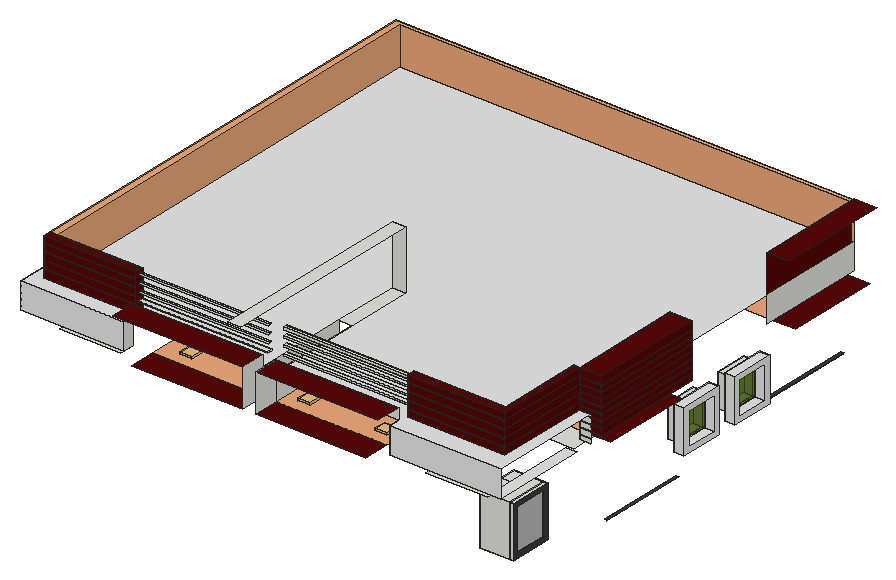
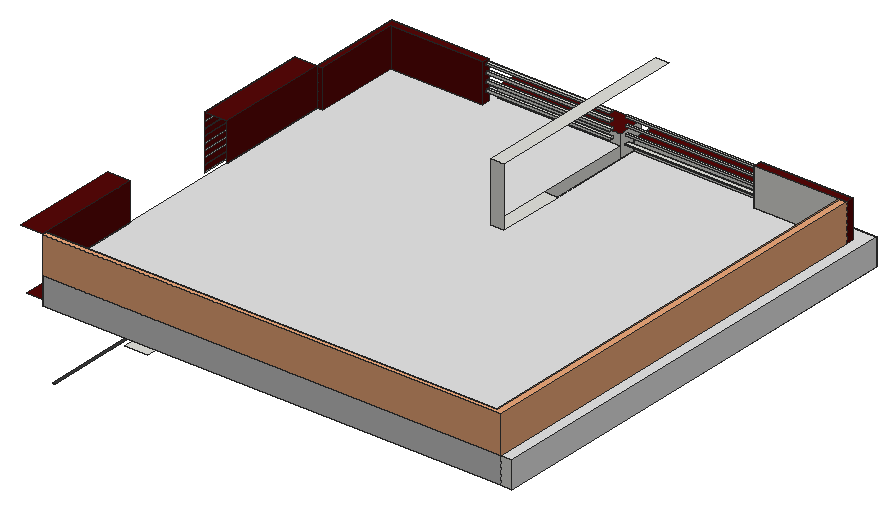
# SketchUp Ruby script. Lengths in inches.
U = 1.inch
M = Sketchup.active_model
def pt(a) = Geom::Point3d.new(a.map { |v| v * U })
def face(e, loops, mat)
  f = e.add_face(loops[0].map { |a| pt(a) })
  loops[1..].each { |l| e.add_face(l.map { |a| pt(a) }).erase! }
  f.material = f.back_material = mat if mat
  f
end
# faces: each face lists its corners as indices into pts; further lists are holes
def faces(e, pts, list, mat = nil) = list.each { |f| face(e, (f[0].is_a?(Array) ? f : [f]).map { |l| l.map { |i| pts[i] } }, mat) }
# xy, xz, yz: faces in a plane at the given z, y or x. An outline is a flat list of corners, or four numbers for a rectangle; further outlines are holes
def ring(l) = l.size == 4 ? [[l[0], l[1]], [l[2], l[1]], [l[2], l[3]], [l[0], l[3]]] : l.each_slice(2).to_a
def flat(e, list, mat, &to3) = list.each { |f| face(e, (f[0].is_a?(Array) ? f : [f]).map { |l| ring(l).map { |u, v| to3.(u, v) } }, mat) }
def xy(e, z, list, mat = nil) = flat(e, list, mat) { |x, y| [x, y, z] }
def xz(e, y, list, mat = nil) = flat(e, list, mat) { |x, z| [x, y, z] }
def yz(e, x, list, mat = nil) = flat(e, list, mat) { |y, z| [x, y, z] }
def lines(e, pts, list) = list.each { |a, b| e.add_line(pt(pts[a]), pt(pts[b])) }
# prism: a flat outline (further loops are holes) pulled along v
def prism(e, loops, v, mat = nil)
  f = face(e, loops, mat); d = Geom::Vector3d.new(v.map { |x| x * U })
  f.pushpull(f.normal.samedirection?(d) ? d.length : -d.length)
end
def box(e, o, s, mat = nil) = prism(e, [[o, [o[0] + s[0], o[1], o[2]], [o[0] + s[0], o[1] + s[1], o[2]], [o[0], o[1] + s[1], o[2]]]], [0, 0, s[2]], mat)
def at(x, y, z, deg = 0) = Geom::Transformation.translation(pt([x, y, z])) * Geom::Transformation.rotation(ORIGIN, Z_AXIS, deg.degrees)
def axes(o, x, y, z) = Geom::Transformation.new([*x, 0, *y, 0, *z, 0, *pt(o).to_a, 1])
def part(name) = M.definitions.add(name)
# library, detail: a bought-in or finely detailed component or shape, given as its bounding box
def library(name, o, s) = part(name).tap { |d| box(d.entities, o, s) }
def detail(e, o, s) = box(e.add_group.entities, o, s)
def put(e, d, t, mat = nil) = e.add_instance(d, t).tap { |i| i.material = mat if mat }
def group(e, t, mat = nil) = e.add_group.tap { |g| g.transformation = t; g.material = mat if mat }.entities
root = M.entities
M.materials.add("Generic").color = [86, 8, 8]
M.materials.add("Generic\#1").color = [236, 168, 122]
M.materials.add("Generic\#4").color = [201, 201, 201]
M.materials.add("Generic\#5").color = [230, 230, 230]
M.materials.add("[Color M07]").color = [58, 58, 58]
M.materials.add("[Mirror 01]").color = [185, 185, 185]
M.materials.add("[Translucent Glass Dark Green]").color = [62, 91, 5]
M.materials["[Translucent Glass Dark Green]"].alpha = 0.5
c1 = part("Group\#3")
xy(c1.entities,0,[[0,0,6,62.6875]],"[Color M07]")
xy(c1.entities,6.1,[[3,6.1,6,56.59]],"[Color M07]")
xy(c1.entities,69.52,[[3,6.1,6,56.59]],"[Color M07]")
xy(c1.entities,75.625,[[0,0,6,62.6875]],"[Color M07]")
xz(c1.entities,0,[[0,0,6,75.625]],"[Color M07]")
xz(c1.entities,6.1,[[3,6.1,6,69.52]],"[Color M07]")
xz(c1.entities,56.59,[[3,6.1,6,69.52]],"[Color M07]")
xz(c1.entities,62.6875,[[0,0,6,75.625]],"[Color M07]")
yz(c1.entities,0,[[0,0,62.6875,75.625]])
yz(c1.entities,3,[[6.1,6.1,56.59,69.52]],"[Mirror 01]")
yz(c1.entities,6,[[[0,0,62.6875,75.625],[6.1,6.1,56.59,69.52]]],"[Color M07]")
c2 = part("Group\#1")
box(c2.entities,[0,0,0],[3,48.3125,48.3125],"[Translucent Glass Dark Green]")
c3 = library("Tlon Light 450 Ceiling 152 006",[-8.86,-8.86,-3.78],[17.72,17.72,3.56])
xy(root,889.17,[[648.625,141.33,698.4375,204.02]])
xy(root,891.34,[[722.32,281.625,725.7,413.625]],"[Color M07]")
xy(root,891.4375,[[688.93,624.8125,693.12,762.8125]],"[Color M07]")
xy(root,902.74,[[698.4375,439.75,713.5625,504.55]])
xy(root,902.74,[[698.4375,533.62,713.5625,598.43]],"Generic\#5")
xy(root,910.99,[[681.875,447.99,698.4375,496.3],[681.875,541.87,698.4375,590.18]])
xy(root,910.99,[[698.4375,447.99,713.5625,496.3],[698.4375,541.87,713.5625,590.18]],"Generic\#5")
xy(root,951.48,[[594.5625,306.16,656.0625,398.23]])
xy(root,959.27,[[205.11,219.4375,322.86,251.5625],[386.36,219.4375,504.11,251.5625]])
xy(root,959.3,[[681.875,447.99,698.4375,496.3],[698.4375,447.99,713.5625,496.3],[681.875,541.87,698.4375,590.18]])
xy(root,959.3,[[698.4375,541.87,713.5625,590.18]],"Generic\#5")
xy(root,964.8,[[648.625,141.33,698.4375,204.02]])
xy(root,966.4,[[563.75,654.65,598.75,746.71]])
xy(root,967.55,[[698.4375,439.75,713.5625,504.55],[698.4375,533.62,713.5625,598.43]],"Generic\#5")
xy(root,980.36,[[44.83,113.625,136.51,130.0625],[589.83,113.625,681.51,158.0625]])
xy(root,997.25,[[183.5625,219.4375,347.9375,255],[367.1875,219.4375,531.5625,255],[16.6875,762.8125,698.4375,774.8125]])
xy(root,997.25,[[183.4375,75.4375,347.9375,113.625],[367.1875,75.4375,531.6875,113.625],[698.4375,281.625,731.4375,413.625],[698.4375,624.8125,731.4375,762.8125]],"Generic")
xy(root,997.25,[[183.5625,113.625,347.9375,219.4375],[367.1875,113.625,531.5625,219.4375],[656.0625,281.625,698.4375,413.625],[598.75,624.8125,698.4375,762.8125]],"Generic\#1")
xy(root,997.25,[[0,96.5625,0,774.8125,16.6875,774.8125,16.6875,113.625,154.5,113.625,154.5,96.5625],[549.5625,96.5625,549.5625,113.625,698.4375,113.625,698.4375,238.3125,715.125,238.3125,715.125,96.5625]],"Generic\#5")
xy(root,1012.8125,[[715.125,263.625,731.4375,263.93],[731.14,263.93,731.4375,431.625]])
xy(root,1013.8125,[[715.125,263.625,731.4375,263.93],[731.14,263.93,731.4375,431.625]])
xy(root,1022.4375,[[715.125,263.625,731.4375,263.93],[731.14,263.93,731.4375,431.625]])
xy(root,1023.4375,[[715.125,263.625,731.4375,263.93],[731.14,263.93,731.4375,431.625]])
xy(root,1032.0625,[[715.125,263.625,731.4375,263.93],[731.14,263.93,731.4375,431.625]])
xy(root,1033.0625,[[715.125,263.625,731.4375,263.93],[731.14,263.93,731.4375,431.625]])
xy(root,1036.5625,[[16.6875,119.0625,154.5,131.0625],[552.85,125.625,552.85,137.625,689.4375,137.625,689.4375,263.625,698.4375,263.625,698.4375,125.625],[16.6875,131.0625,16.6875,774.8125,698.4375,774.8125,698.4375,767.9375,27.5,767.9375,27.5,131.0625],[347.9375,255,367.1875,354.125]])
xy(root,1036.5625,[[0,96.5625,154.5,96.5625,154.5,113.625,347.9375,113.625,347.9375,354.125,367.1875,354.125,367.1875,113.625,549.5625,113.625,549.5625,96.5625,715.125,96.5625,715.125,263.625,698.4375,263.625,698.4375,125.625,552.85,125.625,552.85,137.625,689.4375,137.625,689.4375,263.625,698.4375,263.625,698.4375,767.9375,27.5,767.9375,27.5,131.0625,154.5,131.0625,154.5,119.0625,16.6875,119.0625,16.6875,774.8125,0,774.8125]],"Generic\#5")
xy(root,1041.6875,[[698.4375,263.625,731.4375,263.93],[731.14,263.93,731.4375,431.625]])
xy(root,1042.6875,[[698.4375,263.625,731.4375,263.93],[731.14,263.93,731.4375,431.625]])
xy(root,1046.3125,[[552.85,125.625,698.4375,125.93],[698.14,125.93,698.4375,263.625]])
xy(root,1047.3125,[[552.85,125.625,698.4375,125.93],[698.14,125.93,698.4375,263.625]])
xy(root,1048.5625,[[16.6875,119.0625,154.5,119.36]])
xy(root,1049.5625,[[16.6875,119.0625,154.5,119.36]])
xy(root,1051.13,[[154.5,122.52,347.9375,129.9]])
xy(root,1051.3125,[[698.4375,263.625,731.4375,263.93],[731.14,263.93,731.4375,431.625]])
xy(root,1052.22,[[367.1875,126.95,552.85,132.89]])
xy(root,1052.3125,[[698.4375,263.625,731.4375,263.93],[731.14,263.93,731.4375,431.625]])
xy(root,1052.9375,[[154.5,75.4375,347.9375,113.625],[367.1875,75.4375,549.5625,113.625]],"Generic")
xy(root,1053.13,[[154.5,122.52,347.9375,129.9]])
xy(root,1055.1,[[367.1875,126.95,552.85,132.89]])
xy(root,1058.3125,[[552.85,125.625,698.14,125.93],[698.14,125.625,698.4375,263.625]])
xy(root,1059.3125,[[552.85,125.625,698.14,125.93],[698.14,125.625,698.4375,263.625]])
xy(root,1059.9375,[[16.6875,119.0625,154.5,119.36]])
xy(root,1060.9375,[[16.6875,119.0625,154.5,119.36],[698.4375,263.625,731.4375,263.93],[731.14,263.93,731.4375,431.625]])
xy(root,1061.9375,[[698.4375,263.625,731.4375,263.93],[731.14,263.93,731.4375,431.625]])
xy(root,1063.19,[[154.5,123.11,347.9375,128.18]])
xy(root,1064.22,[[367.1875,126.95,552.85,132.89]])
xy(root,1065.32,[[154.5,123.11,347.9375,128.18]])
xy(root,1067.1,[[367.1875,126.95,552.85,132.89]])
xy(root,1070.3125,[[552.85,125.625,698.4375,125.93],[698.14,125.93,698.4375,263.625]])
xy(root,1070.5625,[[698.4375,263.625,731.4375,263.93],[731.14,263.93,731.4375,431.625]])
xy(root,1071.3125,[[16.6875,119.0625,154.5,119.36],[552.85,125.625,698.4375,125.93],[698.14,125.93,698.4375,263.625]])
xy(root,1071.5625,[[698.4375,263.625,731.4375,263.93],[731.14,263.93,731.4375,431.625]])
xy(root,1072.3125,[[16.6875,119.0625,154.5,119.36]])
xy(root,1075.19,[[154.5,123.11,347.9375,128.18]])
xy(root,1076.22,[[367.1875,126.95,552.85,132.89]])
xy(root,1077.32,[[154.5,123.11,347.9375,128.18]])
xy(root,1079.1,[[367.1875,126.95,552.85,132.89]])
xy(root,1080.1875,[[698.4375,263.625,731.4375,263.93],[731.14,263.93,731.4375,431.625]])
xy(root,1081.1875,[[698.4375,263.625,731.4375,263.93],[731.14,263.93,731.4375,431.625]])
xy(root,1082.3125,[[552.85,125.625,698.14,125.93],[698.14,125.625,698.4375,263.625]])
xy(root,1082.6875,[[16.6875,119.0625,154.5,119.36]])
xy(root,1083.3125,[[552.85,125.625,698.14,125.93],[698.14,125.625,698.4375,263.625]])
xy(root,1083.6875,[[16.6875,119.0625,154.5,119.36]])
xy(root,1087.19,[[154.5,123.11,347.9375,128.18]])
xy(root,1087.4,[[367.1875,126.95,552.85,132.89]])
xy(root,1089.32,[[154.5,123.11,347.9375,128.18]])
xy(root,1090.28,[[367.1875,126.95,552.85,132.89]])
xy(root,1092.375,[[16.6875,119.0625,154.5,131.0625]],"Generic")
xy(root,1092.375,[[16.6875,131.0625,27.5,131.0625,27.5,767.9375,698.4375,767.9375,698.4375,774.8125,16.6875,774.8125]],"Generic\#1")
xy(root,1093.1875,[[552.85,125.625,698.4375,125.625,698.4375,263.625,689.4375,263.625,689.4375,137.625,552.85,137.625],[698.4375,263.625,731.4375,431.625],[698.4375,612.8125,731.4375,774.8125]],"Generic")
xy(root,1124.875,[[347.9375,48.1875,367.1875,354.125]])
xz(root,96.5625,[[0,997.25,154.5,1036.5625],[549.5625,997.25,715.125,1036.5625]],"Generic\#5")
xz(root,113.625,[[154.5,1036.5625,347.9375,1052.9375],[367.1875,1036.5625,549.5625,1052.9375]])
xz(root,119.0625,[[16.6875,1036.5625,154.5,1048.5625],[16.6875,1049.5625,154.5,1059.9375],[16.6875,1060.9375,154.5,1071.3125],[16.6875,1072.3125,154.5,1082.6875],[16.6875,1083.6875,154.5,1092.375]],"Generic")
xz(root,119.36,[[16.6875,1048.5625,154.5,1049.5625],[16.6875,1059.9375,154.5,1060.9375],[16.6875,1071.3125,154.5,1072.3125],[16.6875,1082.6875,154.5,1083.6875]])
xz(root,122.52,[[154.5,1051.13,347.9375,1053.13]])
xz(root,123.11,[[154.5,1063.19,347.9375,1065.32],[154.5,1075.19,347.9375,1077.32],[154.5,1087.19,347.9375,1089.32]])
xz(root,125.625,[[552.85,1036.5625,698.4375,1046.3125],[552.85,1047.3125,698.4375,1058.3125],[552.85,1059.3125,698.4375,1070.3125],[552.85,1071.3125,698.4375,1082.3125],[552.85,1083.3125,698.4375,1093.1875]],"Generic")
xz(root,125.93,[[552.85,1046.3125,698.14,1047.3125],[552.85,1058.3125,698.14,1059.3125],[552.85,1070.3125,698.14,1071.3125],[552.85,1082.3125,698.14,1083.3125]])
xz(root,126.95,[[367.1875,1052.22,552.85,1055.1],[367.1875,1064.22,552.85,1067.1],[367.1875,1076.22,552.85,1079.1],[367.1875,1087.4,552.85,1090.28]])
xz(root,128.18,[[154.5,1063.19,347.9375,1065.32],[154.5,1075.19,347.9375,1077.32],[154.5,1087.19,347.9375,1089.32]])
xz(root,129.9,[[154.5,1051.13,347.9375,1053.13]])
xz(root,131.0625,[[16.6875,1036.5625,27.5,1092.375],[27.5,1036.5625,154.5,1092.375]])
xz(root,132.89,[[367.1875,1052.22,552.85,1055.1],[367.1875,1064.22,552.85,1067.1],[367.1875,1076.22,552.85,1079.1],[367.1875,1087.4,552.85,1090.28]])
xz(root,137.625,[[552.85,1036.5625,689.4375,1093.1875]],"Generic")
xz(root,141.33,[[648.625,889.17,698.4375,964.8]])
xz(root,204.02,[[648.625,889.17,698.4375,964.8]])
xz(root,263.625,[[698.4375,997.25,715.125,1003.1875],[698.4375,1003.1875,715.125,1004.1875],[698.4375,1004.1875,715.125,1012.8125],[698.4375,1012.8125,715.125,1013.8125],[698.4375,1013.8125,715.125,1022.4375],
  [698.4375,1022.4375,715.125,1023.4375],[698.4375,1023.4375,715.125,1032.0625],[698.4375,1032.0625,715.125,1033.0625],[698.4375,1033.0625,715.125,1036.5625],[698.14,1046.3125,698.4375,1047.3125],
  [698.14,1058.3125,698.4375,1059.3125],[698.14,1070.3125,698.4375,1071.3125],[698.14,1082.3125,698.4375,1083.3125]])
xz(root,263.625,[[715.125,1013.8125,731.4375,1022.4375],[715.125,1023.4375,731.4375,1032.0625],[715.125,1033.0625,731.4375,1033.0625,731.4375,1041.6875,698.4375,1041.6875,698.4375,1036.5625,715.125,1036.5625],[689.4375,1036.5625,689.4375,1093.1875,698.4375,1093.1875,698.4375,1083.3125,698.14,1083.3125,698.14,1082.3125,698.4375,1082.3125,698.4375,1071.3125,698.14,1071.3125,698.14,1070.3125,698.4375,1070.3125,698.4375,1059.3125,698.14,1059.3125,698.14,1058.3125,698.4375,1058.3125,698.4375,1047.3125,698.14,1047.3125,698.14,1046.3125,698.4375,1046.3125,698.4375,1036.5625],[698.4375,1042.6875,731.4375,1051.3125],
  [698.4375,1052.3125,731.4375,1060.9375],[698.4375,1061.9375,731.4375,1070.5625],[698.4375,1071.5625,731.4375,1080.1875],[698.4375,1081.1875,731.4375,1093.1875]],"Generic")
xz(root,263.93,[[715.125,1012.8125,731.14,1013.8125],[715.125,1022.4375,731.14,1023.4375],[715.125,1032.0625,731.14,1033.0625],[698.4375,1041.6875,731.14,1042.6875],[698.4375,1051.3125,731.14,1052.3125],
  [698.4375,1060.9375,731.14,1061.9375],[698.4375,1070.5625,731.14,1071.5625],[698.4375,1080.1875,731.14,1081.1875]])
xz(root,354.125,[[347.9375,1036.5625,367.1875,1124.875]])
xz(root,439.75,[[698.4375,902.74,713.5625,967.55]],"Generic\#5")
xz(root,447.99,[[681.875,910.99,698.4375,959.3]])
xz(root,447.99,[[698.4375,910.99,713.5625,959.3]],"Generic\#5")
xz(root,496.3,[[681.875,910.99,698.4375,959.3]])
xz(root,496.3,[[698.4375,910.99,713.5625,959.3]],"Generic\#5")
xz(root,504.55,[[698.4375,902.74,713.5625,967.55]],"Generic\#5")
xz(root,533.62,[[698.4375,902.74,713.5625,967.55]],"Generic\#5")
xz(root,541.87,[[681.875,910.99,698.4375,959.3]])
xz(root,541.87,[[698.4375,910.99,713.5625,959.3]],"Generic\#5")
xz(root,590.18,[[681.875,910.99,698.4375,959.3]])
xz(root,590.18,[[698.4375,910.99,713.5625,959.3]],"Generic\#5")
xz(root,598.43,[[698.4375,902.74,713.5625,967.55]],"Generic\#5")
xz(root,767.9375,[[27.5,1036.5625,698.4375,1092.375]],"Generic\#1")
xz(root,774.8125,[[0,997.25,16.6875,1036.5625]])
xz(root,774.8125,[[16.6875,1036.5625,698.4375,1092.375]],"Generic\#1")
xz(root,774.8125,[[16.6875,997.25,698.4375,1036.5625]],"Generic\#4")
yz(root,0,[[96.5625,997.25,774.8125,1036.5625]],"Generic\#5")
yz(root,16.6875,[[119.0625,1036.5625,119.0625,1048.5625,119.36,1048.5625,119.36,1049.5625,119.0625,1049.5625,119.0625,1059.9375,119.36,1059.9375,119.36,1060.9375,119.0625,1060.9375,119.0625,1071.3125,119.36,1071.3125,119.36,1072.3125,119.0625,1072.3125,119.0625,1082.6875,119.36,1082.6875,119.36,1083.6875,119.0625,1083.6875,119.0625,1092.375,131.0625,1092.375,131.0625,1036.5625]],"Generic")
yz(root,16.6875,[[131.0625,1036.5625,774.8125,1092.375]],"Generic\#1")
yz(root,27.5,[[131.0625,1036.5625,767.9375,1092.375]],"Generic\#1")
yz(root,154.5,[[96.5625,997.25,113.625,1036.5625],[123.11,1063.19,128.18,1065.32],[123.11,1075.19,128.18,1077.32],[123.11,1087.19,128.18,1089.32]])
yz(root,154.5,[[[119.0625,1036.5625,131.0625,1036.5625,131.0625,1092.375,119.0625,1092.375,119.0625,1083.6875,119.36,1083.6875,119.36,1082.6875,119.0625,1082.6875,119.0625,1072.3125,119.36,1072.3125,119.36,1071.3125,119.0625,1071.3125,119.0625,1060.9375,119.36,1060.9375,119.36,1059.9375,119.0625,1059.9375,119.0625,1049.5625,119.36,1049.5625,119.36,1048.5625,119.0625,1048.5625],[122.52,1051.13,129.9,1053.13],[123.11,1087.19,128.18,1089.32],[123.11,1075.19,128.18,1077.32],[123.11,1063.19,128.18,1065.32]]],"Generic")
yz(root,347.9375,[[75.4375,997.25,113.625,1052.9375],[113.625,997.25,255,1036.5625],[122.52,1051.13,129.9,1053.13]])
yz(root,367.1875,[[75.4375,997.25,113.625,1052.9375],[113.625,997.25,255,1036.5625]])
yz(root,549.5625,[[96.5625,997.25,113.625,1036.5625]])
yz(root,552.85,[[126.95,1052.22,132.89,1055.1],[126.95,1064.22,132.89,1067.1],[126.95,1076.22,132.89,1079.1],[126.95,1087.4,132.89,1090.28]])
yz(root,552.85,[[[125.625,1036.5625,125.625,1046.3125,125.93,1046.3125,125.93,1047.3125,125.625,1047.3125,125.625,1058.3125,125.93,1058.3125,125.93,1059.3125,125.625,1059.3125,125.625,1070.3125,125.93,1070.3125,125.93,1071.3125,125.625,1071.3125,125.625,1082.3125,125.93,1082.3125,125.93,1083.3125,125.625,1083.3125,125.625,1093.1875,137.625,1093.1875,137.625,1036.5625],[126.95,1087.4,132.89,1090.28],[126.95,1076.22,132.89,1079.1],[126.95,1064.22,132.89,1067.1],[126.95,1052.22,132.89,1055.1]]],"Generic")
yz(root,648.625,[[141.33,889.17,204.02,964.8]])
yz(root,681.875,[[447.99,910.99,496.3,959.3],[541.87,910.99,590.18,959.3]])
yz(root,689.4375,[[137.625,1036.5625,263.625,1093.1875]],"Generic")
yz(root,698.14,[[125.93,1046.3125,263.625,1047.3125],[125.93,1058.3125,263.625,1059.3125],[125.93,1070.3125,263.625,1071.3125],[125.93,1082.3125,263.625,1083.3125]])
yz(root,698.4375,[[[439.75,902.74,504.55,967.55],[447.99,910.99,496.3,959.3]],[[533.62,902.74,598.43,967.55],[541.87,910.99,590.18,959.3]],[263.625,997.25,431.625,1036.5625],[612.8125,997.25,774.8125,1036.5625],[263.625,1041.6875,263.93,1042.6875],
  [263.625,1051.3125,263.93,1052.3125],[263.625,1060.9375,263.93,1061.9375],[263.625,1070.5625,263.93,1071.3125],[263.625,1071.3125,263.93,1071.5625],[263.625,1080.1875,263.93,1081.1875]])
yz(root,698.4375,[[125.625,1036.5625,263.625,1046.3125],[263.625,1036.5625,263.625,1041.6875,263.93,1041.6875,263.93,1042.6875,263.625,1042.6875,263.625,1051.3125,263.93,1051.3125,263.93,1052.3125,263.625,1052.3125,263.625,1060.9375,263.93,1060.9375,263.93,1061.9375,263.625,1061.9375,263.625,1070.5625,263.93,1070.5625,263.93,1071.5625,263.625,1071.5625,263.625,1080.1875,263.93,1080.1875,263.93,1081.1875,263.625,1081.1875,263.625,1093.1875,431.625,1093.1875,431.625,1036.5625],[612.8125,1036.5625,612.8125,1093.1875,774.8125,1093.1875,774.8125,1092.375,767.9375,1092.375,767.9375,1036.5625],[125.625,1047.3125,263.625,1058.3125],[125.625,1059.3125,263.625,1070.3125],
  [125.625,1071.3125,263.625,1082.3125],[125.625,1083.3125,263.625,1093.1875]],"Generic")
yz(root,713.5625,[[[439.75,902.74,504.55,967.55],[447.99,910.99,496.3,959.3]],[[533.62,902.74,598.43,967.55],[541.87,910.99,590.18,959.3]]],"Generic\#5")
yz(root,715.125,[[263.625,1012.8125,263.93,1013.8125],[263.625,1022.4375,263.93,1023.4375],[263.625,1032.0625,263.93,1033.0625]])
yz(root,731.14,[[263.93,1012.8125,431.625,1013.8125],[263.93,1022.4375,431.625,1023.4375],[263.93,1032.0625,431.625,1033.0625],[263.93,1041.6875,431.625,1042.6875],[263.93,1051.3125,431.625,1052.3125],
  [263.93,1060.9375,431.625,1061.9375],[263.93,1070.5625,431.625,1071.5625],[263.93,1080.1875,431.625,1081.1875]])
yz(root,731.4375,[[263.625,1013.8125,431.625,1022.4375],[263.625,1023.4375,431.625,1032.0625],[263.625,1033.0625,431.625,1041.6875],[263.625,1042.6875,431.625,1051.3125],[263.625,1052.3125,431.625,1060.9375],
  [263.625,1061.9375,431.625,1070.5625],[263.625,1071.5625,431.625,1080.1875],[263.625,1081.1875,431.625,1093.1875]],"Generic")
p = [[691.375,762.8125,889.25],[691.375,624.8125,889.25],[723.6875,413.625,889.25],[723.6875,281.625,889.25],[552.85,129.78,1053.08],[367.1875,129.78,1053.08],
  [552.85,129.78,1065.08],[367.1875,129.78,1065.08],[552.85,129.78,1077.08],[367.1875,129.78,1077.08],[552.85,129.78,1089.08],[367.1875,129.78,1089.08],
  [154.5,125.48,1052.32],[347.9375,125.48,1052.32],[154.5,125.48,1064.32],[347.9375,125.48,1064.32],[154.5,125.48,1076.32],[347.9375,125.48,1076.32],
  [154.5,125.48,1088.32],[347.9375,125.48,1088.32]]
lines(root,p,[[0,1],[2,3],[4,5],[6,7],[8,9],[10,11],[12,13],[14,15],[16,17],[18,19]])
put(root,c1,at(692.4375,141.33,889.17))
put(root,c2,at(695.4375,447.99,910.99))
put(root,c2,at(695.4375,541.87,910.99))
put(root,c3,at(218.03,141.27,999.6875))
put(root,c3,at(321.47,141.27,999.6875))
put(root,c3,at(393.78,141.27,999.6875))
put(root,c3,at(507.78,141.27,999.6875))
